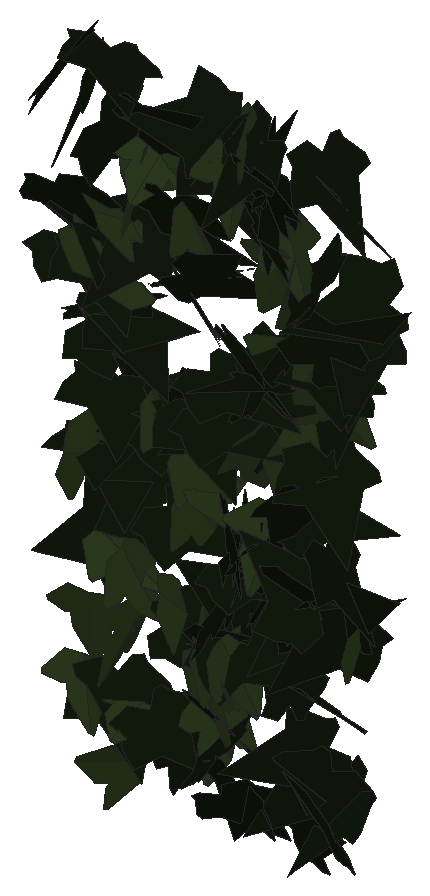
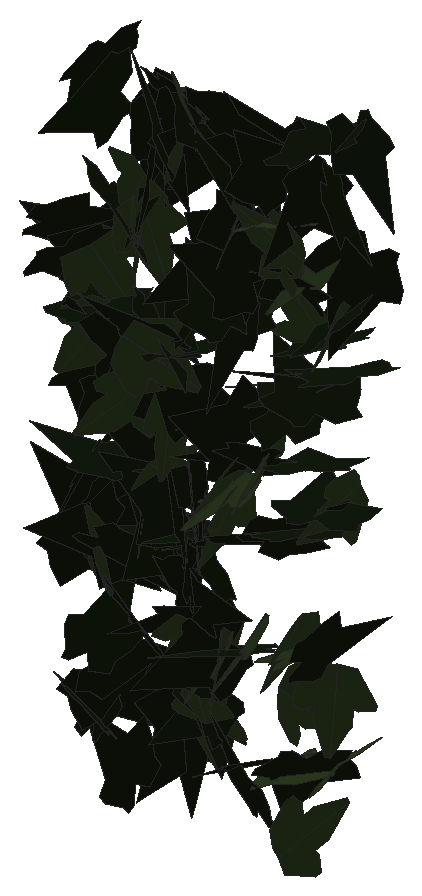
# SketchUp Ruby script. Lengths in inches.
U = 1.inch
M = Sketchup.active_model
def pt(a) = Geom::Point3d.new(a.map { |v| v * U })
def face(e, loops, mat)
  f = e.add_face(loops[0].map { |a| pt(a) })
  loops[1..].each { |l| e.add_face(l.map { |a| pt(a) }).erase! }
  f.material = f.back_material = mat if mat
  f
end
# faces: each face lists its corners as indices into pts; further lists are holes
def faces(e, pts, list, mat = nil) = list.each { |f| face(e, (f[0].is_a?(Array) ? f : [f]).map { |l| l.map { |i| pts[i] } }, mat) }
# xy, xz, yz: faces in a plane at the given z, y or x. An outline is a flat list of corners, or four numbers for a rectangle; further outlines are holes
def ring(l) = l.size == 4 ? [[l[0], l[1]], [l[2], l[1]], [l[2], l[3]], [l[0], l[3]]] : l.each_slice(2).to_a
def flat(e, list, mat, &to3) = list.each { |f| face(e, (f[0].is_a?(Array) ? f : [f]).map { |l| ring(l).map { |u, v| to3.(u, v) } }, mat) }
def xy(e, z, list, mat = nil) = flat(e, list, mat) { |x, y| [x, y, z] }
def xz(e, y, list, mat = nil) = flat(e, list, mat) { |x, z| [x, y, z] }
def yz(e, x, list, mat = nil) = flat(e, list, mat) { |y, z| [x, y, z] }
def lines(e, pts, list) = list.each { |a, b| e.add_line(pt(pts[a]), pt(pts[b])) }
# prism: a flat outline (further loops are holes) pulled along v
def prism(e, loops, v, mat = nil)
  f = face(e, loops, mat); d = Geom::Vector3d.new(v.map { |x| x * U })
  f.pushpull(f.normal.samedirection?(d) ? d.length : -d.length)
end
def box(e, o, s, mat = nil) = prism(e, [[o, [o[0] + s[0], o[1], o[2]], [o[0] + s[0], o[1] + s[1], o[2]], [o[0], o[1] + s[1], o[2]]]], [0, 0, s[2]], mat)
def at(x, y, z, deg = 0) = Geom::Transformation.translation(pt([x, y, z])) * Geom::Transformation.rotation(ORIGIN, Z_AXIS, deg.degrees)
def axes(o, x, y, z) = Geom::Transformation.new([*x, 0, *y, 0, *z, 0, *pt(o).to_a, 1])
def part(name) = M.definitions.add(name)
# library, detail: a bought-in or finely detailed component or shape, given as its bounding box
def library(name, o, s) = part(name).tap { |d| box(d.entities, o, s) }
def detail(e, o, s) = box(e.add_group.entities, o, s)
def put(e, d, t, mat = nil) = e.add_instance(d, t).tap { |i| i.material = mat if mat }
def group(e, t, mat = nil) = e.add_group.tap { |g| g.transformation = t; g.material = mat if mat }.entities
root = M.entities
M.materials.add("efeu1").color = [18, 25, 13]
M.materials.add("efeu2").color = [43, 57, 29]
c1 = part("ivyleaf_10")
p = [[0,0.5,-0.03],[-0.0625,2.02,-0.43],[-0.19,2.01,-0.46],[-0.54,1.05,-0.29],[-0.52,0.625,-0.18],[-0.83,0.76,-0.28],
  [-1.16,0.64,-0.33],[-1.15,0.33,-0.24],[-0.77,-0.39,0.02],[-0.3,-0.51,0.16],[0.04,-0.48,0.23],[-0.02,2.01,-0.4375],
  [-0.06,2.01,-0.43],[0.04,-0.49,0.23],[0.67,-0.49,0.14],[1.38,0.36,-0.2],[1.375,0.51,-0.24],[0.81,0.65,-0.19],
  [0.62,0.59,-0.15],[0.6,1.09,-0.28],[0.5,1.23,-0.31]]
faces(c1.entities,p,[[0,1,2,3,4,5,6,7,8,9,10],[11,12,0,13,14,15,16,17,18,19,20]],"efeu2")
c2 = part("ivyleaf_9")
p = [[1.54,2.16,1.25],[1.36,2.04,1.19],[-0.21,0.99,0.68],[-0.71,1.11,0.82],[-0.85,0.86,0.67],[-0.8,0.17,0.21],
  [-0.9,-0.01,0.1],[-0.67,-0.16,-0.02],[-0.08,-0.08,-0.05],[-0.03,-0.6,-0.4],[0.65,-0.88,-0.66],[0.83,-0.6,-0.49],
  [1.29,-0.42,-0.43],[1.8125,-0.07,-0.26],[1.21,0.44,0.15]]
faces(c2.entities,p,[[0,1,2,3,4,5,6,7,8,9,10,11,12,13,14]],"efeu1")
put(root,c1,axes([51.28,221.8125,227.46],[-0.24526,-0.29556,0.32014],[0.19774,-0.40287,-0.22044],[0.38826,0.01848,0.31451]))
put(root,c2,axes([50.98,221.22,223.5],[0.39992,0.29772,0.03771],[0.02615,0.02803,-0.49853],[-0.29896,0.40072,0.00685]))
put(root,c2,axes([51.03,221.37,223.64],[0.31733,0.09666,-0.37411],[-0.36391,-0.08798,-0.33141],[-0.12989,0.48262,0.01451]))
put(root,c2,axes([51.29,221.65,233.37],[-0.48849,0.00592,-0.10652],[0.10628,-0.01608,-0.48831],[-0.0092,-0.49971,0.01445]))
put(root,c2,axes([51.61,221.32,227],[0.49057,0.09501,-0.01779],[-0.01799,-0.00065,-0.49968],[-0.09498,0.49089,0.00278]))
put(root,c2,axes([52.18,221.63,226.61],[-0.29555,-0.39934,-0.05639],[-0.02031,-0.05509,0.49654],[-0.40279,0.29579,0.01634]))
put(root,c2,axes([48.1,221.45,233.67],[-0.21514,0.4366,-0.11445],[0.05155,-0.10219,-0.48672],[-0.4484,-0.22123,-0.00104]))
put(root,c2,axes([50.77,221.2,225.98],[-0.2961,0.35694,-0.18687],[-0.15393,0.11409,0.46183],[0.37233,0.33103,0.04233]))
put(root,c2,axes([52.39,221.75,223.18],[0.26499,-0.41048,0.10623],[-0.05468,0.09114,0.48857],[-0.42046,-0.27055,0.00341]))
put(root,c2,axes([51.32,221.4,232.98],[0.43847,0.0485,-0.23535],[-0.23428,-0.02261,-0.44114],[-0.05344,0.49713,0.0029]))
put(root,c2,axes([48,221.36,231.7],[0.40726,0.25825,-0.13207],[-0.1113,-0.0711,-0.48224],[-0.26786,0.4222,-0.00043]))
put(root,c2,axes([50.92,221.39,227.45],[0.19005,-0.03896,-0.46083],[-0.45596,0.06755,-0.19375],[0.07736,0.49388,-0.00986]))
put(root,c2,axes([51.37,221.95,229.67],[-0.49286,-0.08355,-0.01057],[0.0819,-0.46087,-0.17576],[0.01963,-0.17498,0.46797]))
put(root,c1,axes([48.375,221.27,227.83],[-0.00637,-0.19291,-0.46124],[0.17396,0.4316,-0.18292],[0.46872,-0.16281,0.06162]))
put(root,c2,axes([48.38,221.95,227.8],[-0.21615,-0.44992,0.02922],[0.3676,-0.19462,-0.27748],[0.26106,-0.09848,0.41491]))
put(root,c2,axes([52.0625,221.55,228.36],[0.02114,0.42868,-0.25649],[-0.03913,-0.25451,-0.4286],[-0.49802,0.03819,0.02279]))
put(root,c1,axes([50.36,221.62,224.84],[-0.38323,0.24917,-0.20261],[0.15521,-0.13246,-0.45647],[-0.28115,-0.41276,0.02418]))
put(root,c2,axes([52.36,221.6,233.5625],[0.12582,-0.42035,-0.23973],[-0.06019,0.23219,-0.43871],[0.48015,0.13925,0.00782]))
put(root,c1,axes([50.66,221.9,233.1875],[-0.14895,0.00158,-0.4773],[0.22651,-0.43987,-0.07214],[-0.42013,-0.23771,0.13032]))
put(root,c2,axes([50.79,221.58,230.21],[0.42952,-0.25592,-0.004],[0.00815,0.02148,-0.49947],[0.25582,0.429,0.02263]))
put(root,c2,axes([52.08,221.95,224.28],[-0.07887,-0.20078,-0.45107],[-0.07844,-0.4459,0.21219],[-0.48747,0.10423,0.03883]))
put(root,c1,axes([50.64,221.84,232.8],[-0.14336,-0.4358,0.19881],[0.22877,-0.24461,-0.37125],[0.42085,-0.01548,0.26953]))
put(root,c2,axes([50.05,221.78,228.77],[0.05391,-0.49415,-0.05393],[0.22028,0.07237,-0.44299],[0.44561,0.02401,0.22551]))
put(root,c2,axes([52.23,221.85,223.99],[0.03474,0.07164,-0.49362],[-0.15503,-0.46876,-0.07895],[-0.47409,0.15853,-0.01036]))
put(root,c1,axes([48.01,221.9375,224.04],[-0.2187,-0.35262,0.27898],[0.3708,-0.31691,-0.10989],[0.25432,0.15882,0.40012]))
put(root,c2,axes([50.56,221.83,226.43],[-0.05003,0.19748,0.45662],[0.05593,-0.45378,0.20238],[0.49434,0.07133,0.02331]))
put(root,c2,axes([50.47,221.62,229.58],[0.27199,-0.40268,-0.11778],[0.25092,0.26862,-0.33895],[0.33625,0.12528,0.3482]))
put(root,c1,axes([48.67,221.56,230.34],[0.46216,0.00264,-0.1908],[0.18936,0.05524,0.45945],[0.02351,-0.49693,0.05006]))
put(root,c2,axes([51.35,221.45,232.2],[0.38966,-0.03048,-0.31182],[-0.2926,0.14252,-0.37957],[0.11202,0.47829,0.09324]))
put(root,c1,axes([51.48,222.02,231.04],[0.00139,0.00998,-0.4999],[0.12389,-0.48432,-0.00932],[-0.48441,-0.12384,-0.00381]))
put(root,c2,axes([50.4,221.64,228.98],[0.27117,-0.37128,-0.19651],[0.2493,0.33049,-0.28041],[0.33811,0.0541,0.36436]))
put(root,c2,axes([50.68,221.41,223.92],[-0.06644,0.43065,0.24521],[-0.13524,0.22226,-0.42698],[-0.47676,-0.12306,0.08694]))
put(root,c2,axes([48.81,222.07,229.07],[-0.20454,-0.30747,0.33709],[0.25672,-0.38294,-0.19352],[0.37717,0.09391,0.31452]))
put(root,c2,axes([50.15,221.43,231.07],[0.3939,0.19785,0.23601],[0.21316,0.10141,-0.44077],[-0.22228,0.44785,-0.00446]))
put(root,c2,axes([50.42,221.75,233.2],[-0.32702,0.08891,0.36763],[-0.35039,0.11177,-0.33872],[-0.14241,-0.47917,-0.0108]))
put(root,c2,axes([49.125,221.78,232.8125],[0.44461,0.09886,-0.20628],[0.19354,0.07777,0.45442],[0.12194,-0.48392,0.03089]))
put(root,c2,axes([52.22,221.83,228.76],[-0.10159,-0.43064,-0.23288],[0.08732,0.21809,-0.44138],[0.48172,-0.13035,0.0309]))
put(root,c2,axes([48.25,221.97,230.52],[-0.0175,-0.49965,-0.00658],[0.2737,-0.00408,-0.41842],[0.41807,-0.01824,0.27365]))
put(root,c2,axes([48.44,221.55,229.71],[0.40273,-0.21099,-0.20806],[0.18405,0.45325,-0.10339],[0.23223,0.00669,0.44275]))
put(root,c2,axes([48.46,222.07,228.59],[-0.15335,-0.4759,-0.00256],[0.29793,-0.0939,-0.39041],[0.37111,-0.12127,0.31236]))
put(root,c1,axes([48.9,221.73,231.35],[0.25634,-0.42436,0.06482],[-0.03113,0.05693,0.49577],[-0.42816,-0.25821,0.00277]))
put(root,c2,axes([49.14,221.95,231.21],[-0.48302,-0.1288,-0.01],[0.00731,0.01141,-0.49982],[0.12898,-0.48299,-0.00914]))
put(root,c2,axes([49.29,221.89,227.11],[-0.32099,-0.35987,-0.13213],[-0.08806,-0.09851,0.48223],[-0.37311,0.33285,-0.00014]))
put(root,c1,axes([48.73,221.47,231.4375],[0.40342,-0.23731,-0.17588],[0.18453,0.43495,-0.1636],[0.23065,0.06709,0.43852]))
put(root,c1,axes([49.91,221.79,231.71],[0.13228,-0.48199,0.0138],[0.28711,0.06724,-0.40379],[0.38739,0.11474,0.29456]))
put(root,c2,axes([52.33,221.73,227.46],[0.27193,-0.35371,-0.2257],[-0.14246,0.17515,-0.44612],[0.39466,0.30694,-0.00552]))
put(root,c2,axes([52.44,221.99,226.25],[0.02143,0.12138,-0.48457],[-0.10755,-0.47252,-0.12312],[-0.48783,0.1095,0.00586]))
put(root,c2,axes([48.7,221.98,229.63],[0.05918,-0.49645,0.00564],[0.27745,0.02836,-0.41499],[0.41173,0.05225,0.27883]))
put(root,c2,axes([52.23,221.61,230.39],[0.00767,-0.02002,0.49954],[0.49663,0.05772,-0.00531],[-0.05746,0.49625,0.02077]))
put(root,c2,axes([48.5625,222.1,227.52],[-0.15335,-0.47589,0.00315],[0.29805,-0.09862,-0.38915],[0.37101,-0.11748,0.31393]))
put(root,c1,axes([50.21,221.67,225.125],[0.2722,-0.4105,-0.08602],[0.25162,0.24187,-0.35803],[0.33556,0.15163,0.33825]))
put(root,c2,axes([50.65,221.66,233.1875],[-0.22438,0.44655,-0.01578],[0.00409,-0.01561,-0.49974],[-0.44681,-0.22439,0.00335]))
put(root,c2,axes([50.84,222.07,228.94],[-0.04286,-0.03591,-0.49686],[-0.16011,-0.47125,0.04787],[-0.47173,0.16321,0.0289]))
put(root,c2,axes([52.03,221.76,233.03],[0.45809,-0.17506,0.09751],[0.09393,-0.02732,-0.49034],[0.17701,0.46755,0.00786]))
put(root,c2,axes([48.33,222.09,233.56],[-0.04055,-0.48011,0.13359],[0.29459,-0.1312,-0.3821],[0.40196,0.04772,0.29352]))
put(root,c2,axes([51.41,221.58,232.45],[0.16466,-0.10217,-0.46092],[-0.39549,0.23674,-0.19376],[0.25783,0.42839,-0.00285]))
put(root,c1,axes([52.27,221.96,230.57],[-0.31538,-0.261,0.28707],[-0.18648,-0.22245,-0.40712],[0.34023,-0.36386,0.04297]))
put(root,c2,axes([51.375,221.71,232.95],[0.14224,0.11544,-0.46523],[-0.45254,-0.12767,-0.17003],[-0.15805,0.46944,0.06816]))
put(root,c2,axes([49.72,221.6875,231.91],[0.34457,0.23306,-0.27741],[-0.23346,-0.14994,-0.41595],[-0.27707,0.41617,0.00549]))
put(root,c2,axes([50.7,221.78,226.66],[0.31632,-0.37782,-0.08479],[0.27723,0.29741,-0.29101],[0.27034,0.1371,0.39765]))
put(root,c1,axes([48.68,222.15,225.01],[0.08772,-0.33902,0.3569],[0.09759,-0.34334,-0.35013],[0.48247,0.13108,0.00594]))
put(root,c2,axes([50.1,221.75,224.35],[0.47665,-0.14206,0.05123],[0.05962,0.02121,-0.49598],[0.13875,0.47892,0.03716]))
put(root,c1,axes([48.79,222.23,223.71],[-0.46585,-0.10067,0.15117],[0.13013,-0.47532,0.08446],[0.1267,0.11804,0.46906]))
put(root,c1,axes([49.11,222.22,232.19],[-0.46512,-0.12828,0.13116],[0.13032,-0.48262,-0.00986],[0.12914,0.02501,0.48239]))
put(root,c2,axes([51.05,221.6,226.87],[0.0819,0.48777,-0.07329],[0.01126,0.07242,0.4946],[0.49312,-0.08267,0.00088]))
put(root,c1,axes([51.43,221.92,231.93],[0.3994,0.0016,0.3008],[0.30076,-0.01006,-0.3993],[0.00477,0.4999,-0.009]))
put(root,c1,axes([48.22,221.81,225.22],[-0.48637,-0.10481,0.0496],[-0.05191,0.00557,-0.49727],[0.10368,-0.48886,-0.0163]))
put(root,c2,axes([50.4,222.16,226.11],[0.0099,0.08734,0.49221],[-0.05728,-0.48887,0.0879],[0.49661,-0.05812,0.00032]))
put(root,c2,axes([52.21,221.65,231.45],[-0.21463,0.3844,0.23699],[-0.15314,0.1849,-0.43859],[-0.42483,-0.26086,0.03837]))
put(root,c1,axes([48.62,222.23,222.76],[-0.10466,-0.12643,-0.47229],[-0.22212,-0.41798,0.16111],[-0.43556,0.24353,0.03133]))
put(root,c2,axes([52.23,221.97,226.43],[0.03781,-0.01692,0.49828],[0.38696,-0.3141,-0.04003],[0.31438,0.38866,-0.01066]))
put(root,c2,axes([51.34,221.61,229.67],[-0.11443,0.39642,0.28242],[-0.17236,0.23831,-0.40435],[-0.45519,-0.18989,0.08212]))
put(root,c1,axes([50.67,221.72,225.3125],[0.05466,0.46865,0.16546],[0.02414,0.16376,-0.4718],[-0.49642,0.05957,-0.00472]))
put(root,c2,axes([50.41,221.875,232.88],[-0.16794,-0.26822,-0.38711],[0.19197,0.33631,-0.3163],[0.43005,-0.25486,-0.00998]))
put(root,c2,axes([47.97,222.22,230.94],[-0.01563,-0.45107,0.21516],[0.152,-0.20936,-0.42786],[0.47608,0.05203,0.14367]))
put(root,c2,axes([52.52,222.08,223.6875],[-0.47514,0.0738,-0.13711],[0.12044,-0.10483,-0.47382],[-0.09868,-0.48328,0.08184]))
put(root,c2,axes([48.61,221.58,232.77],[0.01828,-0.04995,-0.49716],[-0.22178,0.44499,-0.05286],[0.44775,0.22245,-0.00589]))
put(root,c1,axes([49.94,221.8,227.4],[0.05266,-0.44628,-0.21923],[0.21644,0.21905,-0.39392],[0.44764,-0.05342,0.21626]))
put(root,c1,axes([48.28,221.71,230.54],[-0.0063,0.43711,-0.24268],[-0.11246,0.23524,0.42663],[0.48715,0.05996,0.09535]))
put(root,c2,axes([50.98,221.95,232.56],[-0.07175,0.35955,0.33997],[0.07087,-0.33251,0.36662],[0.48972,0.1008,-0.00325]))
put(root,c2,axes([52.01,222.25,229.87],[-0.12394,-0.47317,0.10366],[0.34768,-0.1614,-0.32105],[0.33728,-0.0075,0.36903]))
put(root,c1,axes([51.42,221.9375,231.42],[-0.42566,-0.08226,0.24909],[-0.24129,-0.06348,-0.4333],[0.10291,-0.48908,0.01434]))
put(root,c1,axes([51.36,222.11,226.7],[-0.25596,0.29969,-0.30769],[0.09377,-0.31055,-0.38048],[-0.41916,-0.25248,0.10277]))
put(root,c1,axes([50.28,222,224.17],[0.49988,-0.00909,-0.00571],[-0.00569,0.00094,-0.49997],[0.0091,0.49992,0.00084]))
put(root,c2,axes([50.63,222.14,226.6],[-0.06358,0.13573,0.47701],[0.1148,-0.46382,0.14728],[0.48247,0.12824,0.02781]))
put(root,c2,axes([50.48,221.82,225.46],[0.24411,-0.26929,-0.34336],[0.20618,0.41793,-0.18118],[0.38458,-0.05313,0.31508]))
put(root,c1,axes([50.2,221.71,224.75],[-0.11037,0.3999,-0.2791],[-0.06344,0.27195,0.41475],[0.48352,0.12696,-0.00929]))
put(root,c1,axes([49.86,221.8,228.07],[0.1307,-0.42195,-0.23426],[0.28197,0.26373,-0.31771],[0.39168,-0.04905,0.30689]))
put(root,c1,axes([50.94,221.89,228.62],[-0.09531,-0.46056,-0.16971],[0.03473,0.16612,-0.47032],[0.4896,-0.10144,0.00033]))
put(root,c2,axes([52.03,222.32,224.66],[-0.39209,-0.12968,0.28187],[0.14867,-0.47721,-0.01274],[0.27233,0.07382,0.41278]))
put(root,c2,axes([51.41,222.16,222.75],[0.07542,-0.12024,0.47943],[0.32544,-0.35294,-0.13971],[0.37202,0.33313,0.02503]))
put(root,c2,axes([51.93,221.625,226.26],[0.07167,0.34072,-0.35885],[0.07153,0.35165,0.34817],[0.48964,-0.10124,0.00166]))
put(root,c2,axes([49.53,221.89,227.08],[0.27409,-0.33018,-0.25662],[0.20854,0.37388,-0.25831],[0.36247,0.03457,0.34267]))
put(root,c2,axes([51.9,222.22,226.34],[-0.47249,-0.15264,0.05879],[-0.05957,-0.0068,-0.49639],[0.15234,-0.47608,-0.01176]))
put(root,c2,axes([49.15,221.99,223.79],[0.211,-0.4027,-0.20811],[0.22164,0.29189,-0.34011],[0.39541,0.05127,0.30169]))
put(root,c2,axes([48.23,222.2,229.64],[0.01265,-0.48348,0.12682],[0.48005,-0.02359,-0.13783],[0.13926,0.12524,0.4636]))
put(root,c2,axes([48.46,222.1,224.0625],[-0.12357,-0.4096,-0.25876],[0.12394,0.23143,-0.42553],[0.46837,-0.16931,0.04434]))
put(root,c2,axes([48.01,222.15,233.11],[-0.34703,0.198,-0.30062],[0.26122,-0.14878,-0.39954],[-0.24766,-0.43435,-0.00018]))
put(root,c1,axes([49.21,221.99,228.46],[0.14305,-0.47801,-0.03229],[0.30193,0.11611,-0.38126],[0.37199,0.08958,0.32187]))
put(root,c1,axes([48.7,221.99,225.9375],[0.05885,-0.48383,-0.11156],[0.27491,0.1253,-0.3984],[0.41348,-0.01445,0.28076]))
put(root,c2,axes([51.64,221.8125,224.9375],[-0.39047,0.30621,0.06136],[0.04116,-0.04692,0.49609],[0.30958,0.39247,0.01143]))
put(root,c2,axes([49.45,222.09,231.17],[0.25078,-0.15068,0.40547],[0.36763,-0.17273,-0.29157],[0.22794,0.44436,0.02415]))
put(root,c2,axes([52.46,222.3,230.73],[-0.13968,-0.47882,-0.03494],[0.01809,0.03112,-0.4987],[0.47975,-0.14058,0.00863]))
put(root,c2,axes([50.03,221.85,225.2],[0.44877,0.09111,0.20077],[0.19514,0.04774,-0.45786],[-0.1026,0.48931,0.00729]))
put(root,c2,axes([52.74,222.4,231.08],[-0.3417,-0.13507,0.33911],[-0.26586,-0.2262,-0.35798],[0.25012,-0.42496,0.08276]))
put(root,c2,axes([49.67,222.24,230.51],[0.01209,-0.46265,0.18922],[0.49056,-0.02535,-0.09333],[0.09595,0.18791,0.4533]))
put(root,c1,axes([48.77,222.125,231.89],[0.16702,-0.04725,-0.46891],[0.45488,-0.11395,0.1735],[-0.12326,-0.48454,0.00492]))
put(root,c1,axes([49.97,221.75,227.64],[0.42823,-0.14635,-0.21261],[0.13498,0.47803,-0.05718],[0.22,-0.00843,0.44892]))
put(root,c2,axes([49.19,221.95,228.45],[0.31571,-0.23744,-0.30652],[0.21871,0.43545,-0.11204],[0.32015,-0.06333,0.37881]))
put(root,c1,axes([52.42,221.98,226.23],[0.27829,-0.1636,-0.38182],[-0.29747,0.24229,-0.32063],[0.28994,0.40562,0.03752]))
put(root,c2,axes([47.57,222.17,230.38],[0.18469,-0.45841,-0.07581],[0.29768,0.17938,-0.35946],[0.35676,0.08765,0.33918]))
put(root,c2,axes([51.27,221.69,226.43],[0.05299,0.28185,0.40958],[0.05277,0.40638,-0.28647],[-0.49438,0.07359,0.01332]))
put(root,c1,axes([49.46,221.9,225.62],[0.27467,-0.35247,-0.22432],[0.20921,0.34841,-0.29128],[0.36164,0.06615,0.33888]))
put(root,c2,axes([49.6875,221.95,230.54],[0.39811,-0.01084,-0.3023],[-0.29867,0.06512,-0.39567],[0.04795,0.49562,0.04537]))
put(root,c2,axes([49.35,222.1,223.07],[-0.2094,0.29154,0.34807],[0.20333,-0.28251,0.35895],[0.40597,0.29188,-0.00024]))
put(root,c2,axes([50.68,222.04,225.86],[-0.1892,0.12512,0.44559],[-0.36127,0.26096,-0.22668],[-0.28929,-0.40773,-0.00834]))
put(root,c1,axes([51.99,222.05,229.62],[-0.38705,-0.12087,-0.29254],[0.28368,0.0725,-0.4053],[0.1404,-0.47972,0.01245]))
put(root,c2,axes([49.52,221.87,225.32],[0.46752,-0.11892,-0.13148],[0.06342,0.45847,-0.18916],[0.16554,0.1602,0.44377]))
put(root,c1,axes([51.15,222.38,229.65],[-0.17424,-0.2278,0.40957],[-0.26088,-0.31586,-0.28666],[0.38934,-0.31359,-0.00878]))
put(root,c1,axes([51.52,221.95,228.67],[-0.16922,-0.23136,-0.40968],[0.32473,0.25762,-0.27961],[0.34046,-0.3607,0.06307]))
put(root,c1,axes([48.25,222.21,225.97],[0.01306,-0.49932,-0.02261],[0.47893,0.01898,-0.14234],[0.14301,-0.01794,0.47878]))
put(root,c2,axes([48.09,222.57,225.97],[-0.17755,-0.17371,0.43394],[-0.2629,-0.34669,-0.24635],[0.38647,-0.31565,0.03177]))
put(root,c2,axes([51.68,222.16,227.53],[0.29065,-0.40625,0.02195],[0.38548,0.26635,-0.17454],[0.13012,0.11838,0.46803]))
put(root,c2,axes([52.05,222.32,229.75],[-0.38334,-0.12063,-0.29748],[0.27785,0.10737,-0.40158],[0.16076,-0.4732,-0.01529]))
put(root,c2,axes([49.74,221.87,228.5],[0.01666,-0.0047,0.4997],[0.34545,0.36139,-0.00812],[-0.36109,0.34551,0.01529]))
put(root,c2,axes([51.05,221.94,229.56],[0.49799,0.01091,-0.0434],[0.00347,0.47405,0.15896],[0.04461,-0.15862,0.47207]))
